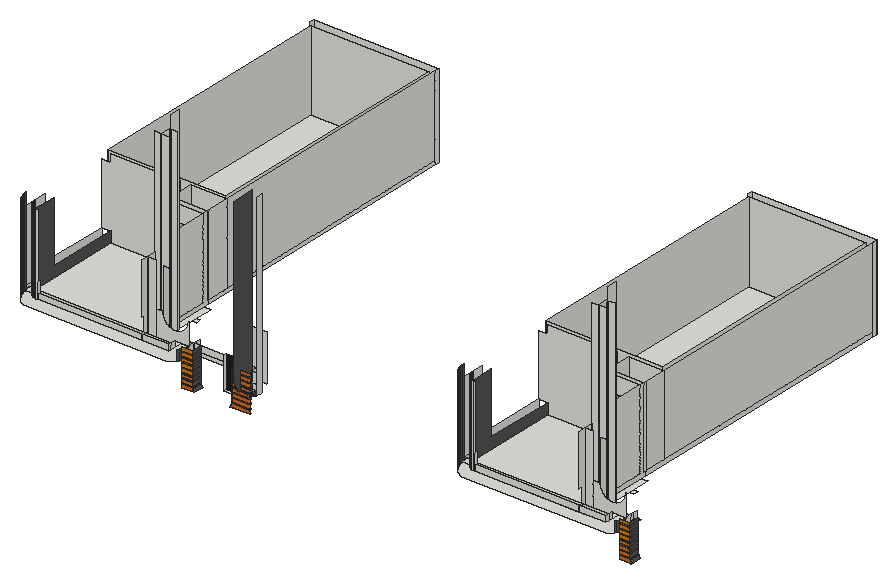
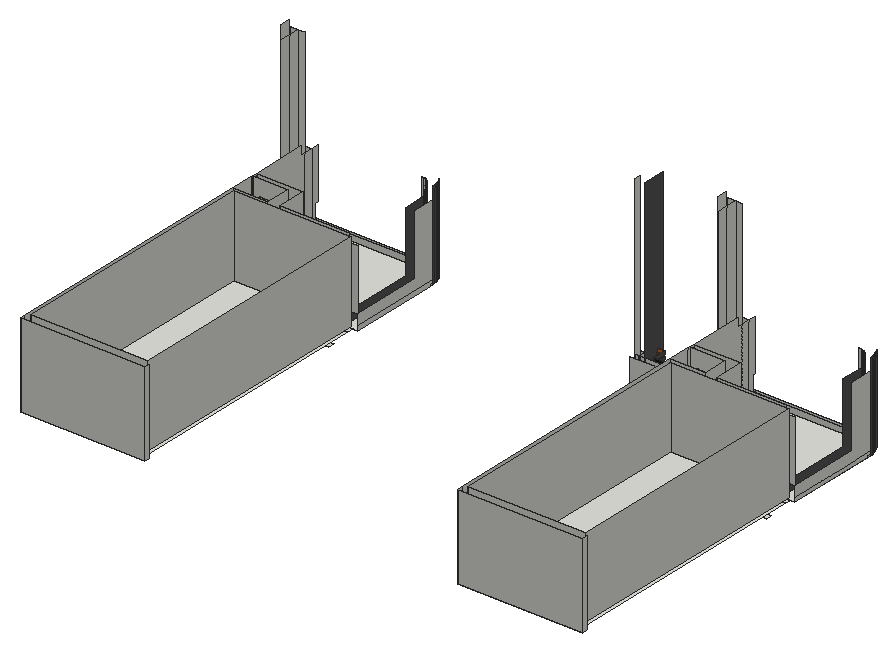
# SketchUp Ruby script. Lengths in inches.
U = 1.inch
M = Sketchup.active_model
def pt(a) = Geom::Point3d.new(a.map { |v| v * U })
def face(e, loops, mat)
  f = e.add_face(loops[0].map { |a| pt(a) })
  loops[1..].each { |l| e.add_face(l.map { |a| pt(a) }).erase! }
  f.material = f.back_material = mat if mat
  f
end
# faces: each face lists its corners as indices into pts; further lists are holes
def faces(e, pts, list, mat = nil) = list.each { |f| face(e, (f[0].is_a?(Array) ? f : [f]).map { |l| l.map { |i| pts[i] } }, mat) }
# xy, xz, yz: faces in a plane at the given z, y or x. An outline is a flat list of corners, or four numbers for a rectangle; further outlines are holes
def ring(l) = l.size == 4 ? [[l[0], l[1]], [l[2], l[1]], [l[2], l[3]], [l[0], l[3]]] : l.each_slice(2).to_a
def flat(e, list, mat, &to3) = list.each { |f| face(e, (f[0].is_a?(Array) ? f : [f]).map { |l| ring(l).map { |u, v| to3.(u, v) } }, mat) }
def xy(e, z, list, mat = nil) = flat(e, list, mat) { |x, y| [x, y, z] }
def xz(e, y, list, mat = nil) = flat(e, list, mat) { |x, z| [x, y, z] }
def yz(e, x, list, mat = nil) = flat(e, list, mat) { |y, z| [x, y, z] }
def lines(e, pts, list) = list.each { |a, b| e.add_line(pt(pts[a]), pt(pts[b])) }
# prism: a flat outline (further loops are holes) pulled along v
def prism(e, loops, v, mat = nil)
  f = face(e, loops, mat); d = Geom::Vector3d.new(v.map { |x| x * U })
  f.pushpull(f.normal.samedirection?(d) ? d.length : -d.length)
end
def box(e, o, s, mat = nil) = prism(e, [[o, [o[0] + s[0], o[1], o[2]], [o[0] + s[0], o[1] + s[1], o[2]], [o[0], o[1] + s[1], o[2]]]], [0, 0, s[2]], mat)
def at(x, y, z, deg = 0) = Geom::Transformation.translation(pt([x, y, z])) * Geom::Transformation.rotation(ORIGIN, Z_AXIS, deg.degrees)
def axes(o, x, y, z) = Geom::Transformation.new([*x, 0, *y, 0, *z, 0, *pt(o).to_a, 1])
def part(name) = M.definitions.add(name)
# library, detail: a bought-in or finely detailed component or shape, given as its bounding box
def library(name, o, s) = part(name).tap { |d| box(d.entities, o, s) }
def detail(e, o, s) = box(e.add_group.entities, o, s)
def put(e, d, t, mat = nil) = e.add_instance(d, t).tap { |i| i.material = mat if mat }
def group(e, t, mat = nil) = e.add_group.tap { |g| g.transformation = t; g.material = mat if mat }.entities
root = M.entities
M.materials.add("[0039_DarkOrange]").color = [219, 120, 0]
M.materials.add("[0041_Chocolate]").color = [210, 105, 30]
M.materials.add("[Color M06]").color = [84, 84, 84]
M.materials.add("[Color M08]").color = [30, 30, 30]
c1 = library("元件\#5",[-4.39,0,0],[5.37,35.83,90.55])
xy(root,90.875,[[820.52,971.36,838.71,972.36],[892.69,971.36,921.96,972.36],[1476.02,971.36,1494.21,972.36]],"[0041_Chocolate]")
xy(root,95.51,[[608.18,1130.875,655.81,1139.4],[1263.68,1130.875,1311.31,1139.4]])
xy(root,95.83,[[820.52,971.36,836.84,972.36],[894.55,971.36,921.96,972.36],[1476.02,971.36,1492.34,972.36]],"[0041_Chocolate]")
xy(root,97.27,[[870.3,986.55,894.74,991.24]])
xy(root,97.9375,[[820.52,971.36,836.56,972.36],[894.83,971.36,921.96,972.36],[1476.02,971.36,1492.06,972.36]],"[0041_Chocolate]")
xy(root,101.1875,[[700.74,1088.75,747.92,1095.9375],[1356.24,1088.75,1403.42,1095.9375]])
xy(root,102.89,[[820.52,971.36,835.91,972.36],[895.48,971.36,921.96,972.36],[1476.02,971.36,1491.41,972.36]],"[0041_Chocolate]")
xy(root,105,[[820.52,971.36,835.91,972.36],[895.48,971.36,921.96,972.36],[1476.02,971.36,1491.41,972.36]],"[0041_Chocolate]")
xy(root,109.9375,[[907.49,990,922.83,993.35]])
xy(root,109.95,[[820.52,971.36,835.91,972.36],[895.48,971.36,921.96,972.36],[1476.02,971.36,1491.41,972.36]],"[0041_Chocolate]")
xy(root,112.0625,[[820.52,971.36,835.91,972.36],[1476.02,971.36,1491.41,972.36]],"[0039_DarkOrange]")
xy(root,112.0625,[[895.48,971.36,921.96,972.36]],"[0041_Chocolate]")
xy(root,117.02,[[820.52,971.36,835.91,972.36],[1476.02,971.36,1491.41,972.36]],"[0039_DarkOrange]")
xy(root,117.02,[[895.48,971.36,921.96,972.36]],"[0041_Chocolate]")
xy(root,119.125,[[820.52,971.36,835.91,972.36],[1476.02,971.36,1491.41,972.36]],"[0039_DarkOrange]")
xy(root,119.125,[[895.48,971.36,921.96,972.36]],"[0041_Chocolate]")
xy(root,124.08,[[820.52,971.36,835.91,972.36],[1476.02,971.36,1491.41,972.36]],"[0039_DarkOrange]")
xy(root,124.08,[[895.48,971.36,921.96,972.36]],"[0041_Chocolate]")
xy(root,126.125,[[592.47,960.52,591.125,960.98,587.53,962.75,584.2,964.98,581.18,967.62,579.44,969.61,578.54,970.63,576.3125,973.96,574.54,977.56,573.25,981.35,572.47,985.28,572.21,989.28,572.21,1130.875,690.69,1130.875,690.69,1088.75,759.32,1088.75,759.32,996.48,769.03,996.48,769.03,1003.71,820.52,1003.71,820.52,996.48,820.02,996.48,820.02,983.34,820.52,983.34,820.3125,980.12,819.68,976.95,818.64,973.89,817.21,970.99,815.42,968.31,813.29,965.88,810.86,963.75,808.17,961.95,805.28,960.52],[1247.97,960.52,1246.625,960.98,1243.03,962.75,1239.7,964.98,1236.68,967.62,1234.94,969.61,1234.04,970.63,1231.8125,973.96,1230.04,977.56,1228.75,981.35,1227.97,985.28,1227.71,989.28,1227.71,1130.875,1346.19,1130.875,1346.19,1088.75,1414.82,1088.75,1414.82,996.48,1424.53,996.48,1424.53,1003.71,1476.02,1003.71,1476.02,996.48,1475.52,996.48,1475.52,983.34,1476.02,983.34,1475.8125,980.12,1475.18,976.95,1474.14,973.89,1472.71,970.99,1470.92,968.31,1468.79,965.88,1466.36,963.75,1463.67,961.95,1460.78,960.52],[820.02,983.34,820.52,993.35],[1475.52,983.34,1476.02,993.35],[820.02,993.35,820.52,996.48],
  [1475.52,993.35,1476.02,996.48],[759.32,996.48,769.03,1003.71],[1414.82,996.48,1424.53,1003.71],[759.32,1003.71,769.03,1088.75],[769.03,1003.71,769.34,1012.23],
  [769.34,1003.71,770.9,1012.23],[770.9,1003.71,780.56,1012.23],[780.56,1003.71,820.52,1012.23],[1414.82,1003.71,1424.53,1088.75],[1424.53,1003.71,1424.84,1012.23],
  [1424.84,1003.71,1426.4,1012.23],[1426.4,1003.71,1436.06,1012.23],[1436.06,1003.71,1476.02,1012.23],[769.03,1012.23,769.34,1027.17],[769.34,1012.23,770.9,1027.17],
  [1424.53,1012.23,1424.84,1027.17],[1424.84,1012.23,1426.4,1027.17],[690.69,1088.75,709.53,1088.75,709.53,1139.4,579.44,1139.4,579.44,1130.875,690.69,1130.875],[709.53,1088.75,759.32,1097.28],[1346.19,1088.75,1365.03,1088.75,1365.03,1139.4,1234.94,1139.4,1234.94,1130.875,1346.19,1130.875],
  [1365.03,1088.75,1414.82,1097.28],[709.53,1097.28,759.32,1521.81],[1365.03,1097.28,1414.82,1521.81],[579.44,1139.4,709.53,1521.81],[1234.94,1139.4,1365.03,1521.81],
  [572.21,1521.81,759.32,1529.04],[1227.71,1521.81,1414.82,1529.04]])
xy(root,126.1875,[[820.52,971.36,835.91,972.36],[1476.02,971.36,1491.41,972.36]],"[0039_DarkOrange]")
xy(root,126.1875,[[895.48,971.36,921.96,972.36]],"[0041_Chocolate]")
xy(root,128.75,[[572.21,985.23,585.21,996.48],[1227.71,985.23,1240.71,996.48]])
xy(root,131.14,[[820.52,971.36,835.91,972.36],[1476.02,971.36,1491.41,972.36]],"[0039_DarkOrange]")
xy(root,131.14,[[895.48,971.36,921.96,972.36]],"[0041_Chocolate]")
xy(root,132.47,[[602.85,972.36,602.85,976.74,759.32,976.74,759.32,1086.875,747.92,1086.875,747.92,1094.0625,700.74,1094.0625,700.74,1086.875,688.99,1086.875,688.99,1130.875,585.93,1130.875,585.93,989.28,586.07,987.07,586.5,984.9,587.21,982.81,588.19,980.82,589.42,978.98,590.88,977.32,592.55,975.86,594.39,974.63,596.37,973.65,598.47,972.9375,600.64,972.5],[602.85,972.36,759.32,976.74],[759.32,972.36,799.9,976.74],[1258.35,972.36,1258.35,976.74,1414.82,976.74,1414.82,1086.875,1403.42,1086.875,1403.42,1094.0625,1356.24,1094.0625,1356.24,1086.875,1344.49,1086.875,1344.49,1130.875,1241.43,1130.875,1241.43,989.28,1241.57,987.07,1242,984.9,1242.71,982.81,1243.69,980.82,1244.92,978.98,1246.38,977.32,1248.05,975.86,1249.89,974.63,1251.87,973.65,1253.97,972.9375,1256.14,972.5],[1258.35,972.36,1414.82,976.74],
  [1414.82,972.36,1455.4,976.74],[759.32,976.74,799.9,983.34],[1414.82,976.74,1455.4,983.34],[759.32,983.34,799.9,1003.71],[1414.82,983.34,1455.4,1003.71],
  [706.57,1094.0625,759.32,1130.875],[1362.07,1094.0625,1414.82,1130.875],[577.71,1136.38,753.81,1516.3],[1233.21,1136.38,1409.31,1516.3]])
xy(root,133.25,[[820.52,971.36,835.91,972.36],[1476.02,971.36,1491.41,972.36]],"[0039_DarkOrange]")
xy(root,133.25,[[895.48,971.36,921.96,972.36]],"[0041_Chocolate]")
xy(root,138.2,[[820.52,971.36,835.91,972.36],[1476.02,971.36,1491.41,972.36]],"[0039_DarkOrange]")
xy(root,138.2,[[895.48,971.36,921.96,972.36]],"[0041_Chocolate]")
xy(root,140.3125,[[820.52,971.36,835.91,972.36],[1476.02,971.36,1491.41,972.36]],"[0039_DarkOrange]")
xy(root,140.3125,[[895.48,971.36,921.96,972.36]],"[0041_Chocolate]")
xz(root,971.36,[[820.52,112.0625,835.91,117.02],[1476.02,112.0625,1491.41,117.02],[820.52,119.125,835.91,124.08],[1476.02,119.125,1491.41,124.08],[820.52,126.1875,835.91,131.14],
  [1476.02,126.1875,1491.41,131.14],[820.52,133.25,835.91,138.2],[1476.02,133.25,1491.41,138.2],[820.52,140.3125,835.91,145.27],[1476.02,140.3125,1491.41,145.27]],"[0039_DarkOrange]")
xz(root,971.36,[[820.52,90.875,838.71,90.875,836.92,95.18,836.84,95.83,820.52,95.83],[892.69,90.875,921.96,90.875,921.96,95.83,894.55,95.83,894.47,95.18],[1476.02,90.875,1494.21,90.875,1492.42,95.18,1492.34,95.83,1476.02,95.83],[820.52,97.9375,836.56,97.9375,835.91,102.89,820.52,102.89],[894.83,97.9375,921.96,97.9375,921.96,102.89,895.48,102.89],
  [1476.02,97.9375,1492.06,97.9375,1491.41,102.89,1476.02,102.89],[820.52,105,835.91,109.95],[895.48,105,921.96,109.95],[1476.02,105,1491.41,109.95],[895.48,112.0625,921.96,117.02],
  [895.48,119.125,921.96,124.08],[895.48,126.1875,921.96,131.14],[895.48,133.25,921.96,138.2],[895.48,140.3125,921.96,145.27]],"[0041_Chocolate]")
xz(root,972.36,[[602.85,132.47,759.32,141.26],[759.32,132.47,799.9,141.26],[1258.35,132.47,1414.82,141.26],[1414.82,132.47,1455.4,141.26]])
xz(root,972.36,[[820.52,117.02,835.91,119.125],[1476.02,117.02,1491.41,119.125],[820.52,124.08,835.91,126.1875],[1476.02,124.08,1491.41,126.1875],[820.52,131.14,835.91,133.25],
  [1476.02,131.14,1491.41,133.25],[820.52,138.2,835.91,140.3125],[1476.02,138.2,1491.41,140.3125]],"[0039_DarkOrange]")
xz(root,972.36,[[820.52,95.83,836.84,95.83,836.56,97.9375,820.52,97.9375],[894.55,95.83,921.96,95.83,921.96,97.9375,894.83,97.9375],[1476.02,95.83,1492.34,95.83,1492.06,97.9375,1476.02,97.9375],[820.52,102.89,835.91,105],[895.48,102.89,921.96,105],
  [1476.02,102.89,1491.41,105],[820.52,109.95,835.91,112.0625],[895.48,109.95,921.96,112.0625],[1476.02,109.95,1491.41,112.0625],[895.48,117.02,921.96,119.125],
  [895.48,124.08,921.96,126.1875],[895.48,131.14,921.96,133.25],[895.48,138.2,921.96,140.3125]],"[0041_Chocolate]")
xz(root,976.74,[[602.85,132.47,799.9,141.26],[1258.35,132.47,1455.4,141.26]])
xz(root,983.34,[[915.16,126.125,916.04,141.26],[916.04,126.125,921.96,141.26],[759.32,132.47,770.9,240.16],[770.9,132.47,799.9,132.47,799.9,141.26,820.52,141.26,820.52,174.51,820.5,173.46,820.41,172.42,820.28,171.38,820.09,170.36,819.84,169.34,819.55,168.33,819.2,167.35,818.8,166.38,818.35,165.4375,817.85,164.52,817.3,163.625,816.71,162.76,816.07,161.93,815.39,161.14,814.67,160.38,813.91,159.66,813.12,158.98,812.29,158.34,811.42,157.75,810.53,157.2,809.61,156.7,808.67,156.25,807.7,155.85,806.71,155.5,805.71,155.21,804.69,154.96,803.67,154.77,802.63,154.64,801.59,154.55,800.54,154.53,799.49,154.55,798.45,154.64,797.41,154.77,796.38,154.96,795.37,155.21,794.36,155.5,793.38,155.85,792.41,156.25,791.47,156.7,790.55,157.2,789.66,157.75,788.79,158.34,787.96,158.98,787.17,159.66,786.41,160.38,785.6875,161.14,785.01,161.93,784.37,162.76,783.78,163.625,783.23,164.52,782.73,165.4375,782.28,166.38,781.88,167.35,781.53,168.33,781.24,169.34,780.99,170.36,780.8,171.38,780.66,172.42,780.58,173.46,780.56,174.51,770.9,174.51],[1414.82,132.47,1426.4,240.16],
  [1426.4,132.47,1455.4,132.47,1455.4,141.26,1476.02,141.26,1476.02,174.51,1476,173.46,1475.91,172.42,1475.78,171.38,1475.59,170.36,1475.34,169.34,1475.05,168.33,1474.7,167.35,1474.3,166.38,1473.85,165.4375,1473.35,164.52,1472.8,163.625,1472.21,162.76,1471.57,161.93,1470.89,161.14,1470.17,160.38,1469.41,159.66,1468.62,158.98,1467.79,158.34,1466.92,157.75,1466.03,157.2,1465.11,156.7,1464.17,156.25,1463.2,155.85,1462.21,155.5,1461.21,155.21,1460.19,154.96,1459.17,154.77,1458.13,154.64,1457.09,154.55,1456.04,154.53,1454.99,154.55,1453.95,154.64,1452.91,154.77,1451.88,154.96,1450.87,155.21,1449.86,155.5,1448.88,155.85,1447.91,156.25,1446.97,156.7,1446.05,157.2,1445.16,157.75,1444.29,158.34,1443.46,158.98,1442.67,159.66,1441.91,160.38,1441.1875,161.14,1440.51,161.93,1439.87,162.76,1439.28,163.625,1438.73,164.52,1438.23,165.4375,1437.78,166.38,1437.38,167.35,1437.03,168.33,1436.74,169.34,1436.49,170.36,1436.3,171.38,1436.16,172.42,1436.08,173.46,1436.06,174.51,1426.4,174.51]])
xz(root,986.55,[[894.74,97.27,895.48,97.27,895.48,102.89,894.83,97.9375]])
xz(root,991.24,[[870.3,97.27,894.74,97.27,894.83,97.9375,895.48,102.89,895.48,145.27,870.3,145.27]],"[Color M08]")
xz(root,993.35,[[820.02,95.62,820.52,126.125],[1475.52,95.62,1476.02,126.125],[907.49,109.9375,915.16,126.125],[915.16,109.9375,916.04,126.125],[916.04,109.9375,922.83,126.125],
  [820.52,126.125,907.49,132.47],[907.49,126.125,915.16,132.47],[915.16,126.125,916.04,132.47],[916.04,126.125,922.83,132.47],[820.52,132.47,907.49,141.26],
  [907.49,132.47,915.16,141.26],[915.16,132.47,916.04,141.26],[916.04,132.47,922.83,141.26]])
xz(root,996.48,[[759.32,126.125,769.03,402.64],[769.03,126.125,770.9,126.125,770.9,226.8,780.56,226.8,780.56,402.64,769.03,402.64],[1414.82,126.125,1424.53,402.64],[1424.53,126.125,1426.4,126.125,1426.4,226.8,1436.06,226.8,1436.06,402.64,1424.53,402.64]])
xz(root,1003.71,[[759.32,126.125,820.52,132.47],[1414.82,126.125,1476.02,132.47]])
xz(root,1012.23,[[769.03,126.125,770.9,402.64],[770.9,126.125,780.56,402.64],[1424.53,126.125,1426.4,402.64],[1426.4,126.125,1436.06,402.64]])
xz(root,1034.04,[[861.07,96.14,897.76,165.14]])
xz(root,1086.875,[[688.99,132.47,700.74,132.47,700.74,227.53,747.92,227.53,747.92,132.47,759.32,132.47,759.32,252.47,688.99,252.47],[1344.49,132.47,1356.24,132.47,1356.24,227.53,1403.42,227.53,1403.42,132.47,1414.82,132.47,1414.82,252.47,1344.49,252.47]])
xz(root,1094.0625,[[700.74,132.47,706.57,227.53],[706.57,132.47,747.92,227.53],[747.92,132.47,747.92,227.53,706.57,227.53,706.57,252.47,759.32,252.47,759.32,132.47],[1356.24,132.47,1362.07,227.53],[1362.07,132.47,1403.42,227.53],
  [1403.42,132.47,1403.42,227.53,1362.07,227.53,1362.07,252.47,1414.82,252.47,1414.82,132.47]])
xz(root,1130.875,[[585.93,132.47,688.99,132.47,688.99,252.47,585.93,252.47,585.93,240.16,572.21,240.16,572.21,148.66,585.93,148.66],[706.57,132.47,759.32,252.47],[1241.43,132.47,1344.49,132.47,1344.49,252.47,1241.43,252.47,1241.43,240.16,1227.71,240.16,1227.71,148.66,1241.43,148.66],[1362.07,132.47,1414.82,252.47]])
xz(root,1136.38,[[577.71,132.47,753.81,252.47],[1233.21,132.47,1409.31,252.47]])
xz(root,1516.3,[[577.71,132.47,753.81,252.47],[1233.21,132.47,1409.31,252.47]])
xz(root,1529.04,[[572.21,126.125,759.32,252.47],[1227.71,126.125,1414.82,252.47]])
yz(root,572.21,[[989.28,126.125,996.48,128.75],[996.48,126.125,996.48,128.75,989.28,128.75,989.28,132.47,1130.875,132.47,1130.875,126.125],[1521.81,126.125,1529.04,252.47],[989.28,132.47,989.28,240.16,1024.22,240.16,1024.22,148.66,1130.875,148.66,1130.875,132.47]])
yz(root,577.71,[[1136.38,132.47,1516.3,252.47]])
yz(root,585.93,[[989.28,132.47,1130.875,132.47,1130.875,148.66,1024.22,148.66,1024.22,240.16,989.28,240.16]],"[Color M06]")
yz(root,602.85,[[972.36,132.47,976.74,155.39]])
yz(root,688.99,[[1086.875,132.47,1130.875,252.47]])
yz(root,700.74,[[1086.875,132.47,1094.0625,227.53]])
yz(root,706.57,[[1094.0625,132.47,1130.875,252.47]])
yz(root,747.92,[[1086.875,132.47,1094.0625,227.53]])
yz(root,753.81,[[1136.38,132.47,1516.3,252.47]])
yz(root,759.32,[[1003.71,126.125,1003.71,132.47,1086.875,132.47,1086.875,252.47,1094.0625,252.47,1094.0625,132.47,1097.28,132.47,1097.28,126.125],[1097.28,126.125,1521.81,132.47],[1521.81,126.125,1529.04,252.47],[972.36,132.47,972.36,141.26,976.74,141.26,976.74,163.7,972.36,163.7,972.36,240.16,983.34,240.16,983.34,132.47],[983.34,132.47,996.48,240.16],
  [996.48,132.47,996.48,240.16,1003.71,240.16,1003.71,252.47,1086.875,252.47,1086.875,132.47],[1094.0625,132.47,1097.28,252.47],[1097.28,132.47,1130.875,252.47],[1130.875,132.47,1521.81,252.47]])
yz(root,769.03,[[996.48,126.125,1012.23,402.64],[1012.23,126.125,1028.46,402.64]])
yz(root,770.9,[[1012.23,126.125,1027.17,421.25]])
yz(root,799.9,[[972.36,132.47,976.74,141.26],[976.74,132.47,983.34,141.26]])
yz(root,820.02,[[993.35,95.62,996.48,126.125]])
yz(root,820.52,[[983.34,126.125,993.35,141.26],[993.35,126.125,996.48,132.47],[996.48,126.125,1003.71,132.47],[993.35,132.47,996.48,141.26],[996.48,132.47,1003.71,141.26]])
yz(root,835.91,[[972.36,102.89,986.55,105],[971.36,105,986.55,109.95],[972.36,109.95,986.55,112.0625],[971.36,112.0625,986.55,117.02],[972.36,117.02,986.55,119.125],
  [971.36,119.125,986.55,124.08],[972.36,124.08,986.55,126.1875],[971.36,126.1875,986.55,131.14],[972.36,131.14,986.55,133.25],[971.36,133.25,986.55,138.2],
  [972.36,138.2,986.55,140.3125],[971.36,140.3125,986.55,145.27]],"[Color M06]")
yz(root,870.3,[[986.55,97.27,991.24,145.27]])
yz(root,895.48,[[972.36,102.89,991.24,105],[971.36,105,991.24,109.95],[972.36,109.95,991.24,112.0625],[971.36,112.0625,991.24,117.02],[972.36,117.02,991.24,119.125],
  [971.36,119.125,991.24,124.08],[972.36,124.08,991.24,126.1875],[971.36,126.1875,991.24,131.14],[972.36,131.14,991.24,133.25],[971.36,133.25,991.24,138.2],
  [972.36,138.2,991.24,140.3125],[971.36,140.3125,991.24,145.27]],"[Color M06]")
yz(root,907.49,[[990,109.9375,985.91,110.21,981.89,111.01,978,112.32,974.32,114.14,970.91,116.42,967.83,119.12,965.125,122.21,962.85,125.62,961.03,129.3,959.71,133.18,958.91,137.2,958.64,141.3,958.64,376.875,993.35,376.875,993.35,109.9375]],"[Color M06]")
yz(root,915.16,[[983.34,126.125,993.35,141.26]])
yz(root,922.83,[[990,109.9375,993.35,109.9375,993.35,376.875,983.34,376.875,983.34,110.72,985.91,110.21]])
yz(root,1227.71,[[989.28,126.125,996.48,128.75],[996.48,126.125,996.48,128.75,989.28,128.75,989.28,132.47,1130.875,132.47,1130.875,126.125],[1521.81,126.125,1529.04,252.47],[989.28,132.47,989.28,240.16,1024.22,240.16,1024.22,148.66,1130.875,148.66,1130.875,132.47]])
yz(root,1233.21,[[1136.38,132.47,1516.3,252.47]])
yz(root,1241.43,[[989.28,132.47,1130.875,132.47,1130.875,148.66,1024.22,148.66,1024.22,240.16,989.28,240.16]],"[Color M06]")
yz(root,1258.35,[[972.36,132.47,976.74,155.39]])
yz(root,1344.49,[[1086.875,132.47,1130.875,252.47]])
yz(root,1356.24,[[1086.875,132.47,1094.0625,227.53]])
yz(root,1362.07,[[1094.0625,132.47,1130.875,252.47]])
yz(root,1403.42,[[1086.875,132.47,1094.0625,227.53]])
yz(root,1409.31,[[1136.38,132.47,1516.3,252.47]])
yz(root,1414.82,[[1003.71,126.125,1003.71,132.47,1086.875,132.47,1086.875,252.47,1094.0625,252.47,1094.0625,132.47,1097.28,132.47,1097.28,126.125],[1097.28,126.125,1521.81,132.47],[1521.81,126.125,1529.04,252.47],[972.36,132.47,972.36,141.26,976.74,141.26,976.74,163.7,972.36,163.7,972.36,240.16,983.34,240.16,983.34,132.47],[983.34,132.47,996.48,240.16],
  [996.48,132.47,996.48,240.16,1003.71,240.16,1003.71,252.47,1086.875,252.47,1086.875,132.47],[1094.0625,132.47,1097.28,252.47],[1097.28,132.47,1130.875,252.47],[1130.875,132.47,1521.81,252.47]])
yz(root,1424.53,[[996.48,126.125,1012.23,402.64],[1012.23,126.125,1028.46,402.64]])
yz(root,1426.4,[[1012.23,126.125,1027.17,421.25]])
yz(root,1455.4,[[972.36,132.47,976.74,141.26],[976.74,132.47,983.34,141.26]])
yz(root,1475.52,[[993.35,95.62,996.48,126.125]])
yz(root,1476.02,[[983.34,126.125,993.35,141.26],[993.35,126.125,996.48,132.47],[996.48,126.125,1003.71,132.47],[993.35,132.47,996.48,141.26],[996.48,132.47,1003.71,141.26]])
yz(root,1491.41,[[972.36,102.89,986.55,105],[971.36,105,986.55,109.95],[972.36,109.95,986.55,112.0625],[971.36,112.0625,986.55,117.02],[972.36,117.02,986.55,119.125],
  [971.36,119.125,986.55,124.08],[972.36,124.08,986.55,126.1875],[971.36,126.1875,986.55,131.14],[972.36,131.14,986.55,133.25],[971.36,133.25,986.55,138.2],
  [972.36,138.2,986.55,140.3125],[971.36,140.3125,986.55,145.27]],"[Color M06]")
p = [[836.92,986.55,95.18],[836.92,971.36,95.18],[838.71,971.36,90.875],[838.71,972.36,90.875],[838.71,986.55,90.875],[892.69,986.55,90.875],
  [892.69,972.36,90.875],[892.69,971.36,90.875],[894.47,971.36,95.18],[894.47,986.55,95.18],[1492.42,986.55,95.18],[1492.42,971.36,95.18],
  [1494.21,971.36,90.875],[1494.21,972.36,90.875],[1494.21,986.55,90.875],[836.84,986.55,95.83],[836.84,972.36,95.83],[836.84,971.36,95.83],
  [894.55,971.36,95.83],[894.55,972.36,95.83],[894.55,986.55,95.83],[1492.34,986.55,95.83],[1492.34,972.36,95.83],[1492.34,971.36,95.83],
  [836.56,972.36,97.9375],[836.56,986.55,97.9375],[894.83,972.36,97.9375],[894.83,986.55,97.9375],[894.74,986.55,97.27],[1492.06,972.36,97.9375],
  [1492.06,986.55,97.9375],[894.83,991.24,97.9375],[894.74,991.24,97.27],[835.91,986.55,102.89],[835.91,972.36,102.89],[835.91,971.36,102.89],
  [836.56,971.36,97.9375],[894.83,971.36,97.9375],[895.48,971.36,102.89],[895.48,972.36,102.89],[895.48,986.55,102.89],[1491.41,986.55,102.89],
  [1491.41,972.36,102.89],[1491.41,971.36,102.89],[1492.06,971.36,97.9375],[895.48,991.24,102.89],[922.83,990,109.9375],[922.83,985.91,110.21],
  [907.49,985.91,110.21],[907.49,990,109.9375],[922.83,983.34,110.72],[922.83,981.89,111.01],[907.49,981.89,111.01],[922.83,978,112.32],
  [907.49,978,112.32],[922.83,974.32,114.14],[907.49,974.32,114.14],[922.83,970.91,116.42],[907.49,970.91,116.42],[817.21,970.99,141.26],
  [815.42,968.31,141.26],[815.42,968.31,126.125],[817.21,970.99,126.125],[1472.71,970.99,141.26],[1470.92,968.31,141.26],[1470.92,968.31,126.125],
  [1472.71,970.99,126.125],[576.3125,973.96,258.13],[576.3125,973.96,126.125],[578.54,970.63,126.125],[578.54,970.63,258.13],[1231.8125,973.96,258.13],
  [1231.8125,973.96,126.125],[1234.04,970.63,126.125],[1234.04,970.63,258.13],[817.89,972.36,141.26],[818.64,973.89,126.125],[818.64,973.89,141.26],
  [1473.39,972.36,141.26],[1474.14,973.89,126.125],[1474.14,973.89,141.26],[819.68,976.95,141.26],[819.68,976.95,126.125],[1475.18,976.95,141.26],
  [1475.18,976.95,126.125],[574.54,977.56,258.13],[574.54,977.56,126.125],[1230.04,977.56,258.13],[1230.04,977.56,126.125],[820.3125,980.12,141.26],
  [820.3125,980.12,126.125],[1475.8125,980.12,141.26],[1475.8125,980.12,126.125],[573.25,981.35,258.13],[573.25,981.35,126.125],[1228.75,981.35,258.13],
  [1228.75,981.35,126.125],[820.52,983.34,141.26],[820.52,983.34,126.125],[1476.02,983.34,141.26],[1476.02,983.34,126.125],[572.47,985.28,258.13],
  [572.47,985.28,126.125],[1227.97,985.28,258.13],[1227.97,985.28,126.125],[572.21,989.28,240.16],[572.21,989.28,132.47],[572.21,989.28,128.75],
  [572.21,989.28,126.125],[572.21,989.28,258.13],[1227.71,989.28,240.16],[1227.71,989.28,132.47],[1227.71,989.28,128.75],[1227.71,989.28,126.125],
  [1227.71,989.28,258.13],[600.64,972.5,252.47],[602.85,972.36,252.47],[602.85,972.36,240.16],[602.85,972.36,164.97],[602.85,972.36,163.7],
  [602.85,972.36,155.39],[602.85,972.36,141.26],[602.85,972.36,132.47],[600.64,972.5,132.47],[1256.14,972.5,252.47],[1258.35,972.36,252.47],
  [1258.35,972.36,240.16],[1258.35,972.36,164.97],[1258.35,972.36,163.7],[1258.35,972.36,155.39],[1258.35,972.36,141.26],[1258.35,972.36,132.47],
  [1256.14,972.5,132.47],[598.47,972.9375,252.47],[598.47,972.9375,132.47],[1253.97,972.9375,252.47],[1253.97,972.9375,132.47],[596.37,973.65,252.47],
  [596.37,973.65,132.47],[1251.87,973.65,252.47],[1251.87,973.65,132.47],[594.39,974.63,252.47],[594.39,974.63,132.47],[1249.89,974.63,252.47],
  [1249.89,974.63,132.47],[592.55,975.86,252.47],[592.55,975.86,132.47],[1248.05,975.86,252.47],[1248.05,975.86,132.47],[590.88,977.32,252.47],
  [590.88,977.32,132.47],[1246.38,977.32,252.47],[1246.38,977.32,132.47],[589.42,978.98,252.47],[589.42,978.98,132.47],[1244.92,978.98,252.47],
  [1244.92,978.98,132.47],[588.19,980.82,252.47],[588.19,980.82,132.47],[1243.69,980.82,252.47],[1243.69,980.82,132.47],[587.21,982.81,252.47],
  [587.21,982.81,132.47],[1242.71,982.81,252.47],[1242.71,982.81,132.47],[586.5,984.9,252.47],[586.5,984.9,132.47],[1242,984.9,252.47],
  [1242,984.9,132.47],[586.07,987.07,252.47],[586.07,987.07,132.47],[1241.57,987.07,252.47],[1241.57,987.07,132.47],[585.93,989.28,252.47],
  [585.93,989.28,132.47],[585.93,989.28,240.16],[1241.43,989.28,252.47],[1241.43,989.28,132.47],[1241.43,989.28,240.16],[897.76,1012.23,96.14],
  [897.76,1034.04,96.14],[861.07,1012.23,96.14],[861.07,1034.04,96.14]]
faces(root,p,[[0,1,2,3,4],[5,6,7,8,9],[10,11,12,13,14],[15,16,17,1,0],[9,8,18,19,20],[21,22,23,11,10],[24,16,15,25],[19,26,27,28,20],
  [29,22,21,30],[33,34,35,36,24,25],[27,26,37,38,39,40],[41,42,43,44,29,30],[27,40,45,31],[46,47,48,49],[50,51,52,48,47],[51,53,54,52],
  [53,55,56,54],[55,57,58,56],[59,60,61,62],[63,64,65,66],[67,68,69,70],[71,72,73,74],[75,59,62,76,77],[78,63,66,79,80],
  [81,77,76,82],[83,80,79,84],[85,86,68,67],[87,88,72,71],[89,81,82,90],[91,83,84,92],[93,94,86,85],[95,96,88,87],
  [97,89,90,98],[99,91,92,100],[101,102,94,93],[103,104,96,95],[105,106,107,108,102,101,109],[110,111,112,113,104,103,114]],"[Color M06]")
faces(root,p,[[28,27,31,32],[115,116,117,118,119,120,121,122,123],[124,125,126,127,128,129,130,131,132],[133,115,123,134],[135,124,132,136],[137,133,134,138],[139,135,136,140],[141,137,138,142],
  [143,139,140,144],[145,141,142,146],[147,143,144,148],[149,145,146,150],[151,147,148,152],[153,149,150,154],[155,151,152,156],[157,153,154,158],
  [159,155,156,160],[161,157,158,162],[163,159,160,164],[165,161,162,166],[167,163,164,168],[169,165,166,170],[171,167,168,172],[173,169,170,174,175],
  [176,171,172,177,178]])
lines(root,p,[[179,180],[181,182]])
put(root,c1,axes([700.74,1087.03,132.47],[0,-1.05,0],[1.302,0,0],[0,0,1.05]))
put(root,c1,axes([1356.24,1087.03,132.47],[0,-1.05,0],[1.302,0,0],[0,0,1.05]))
